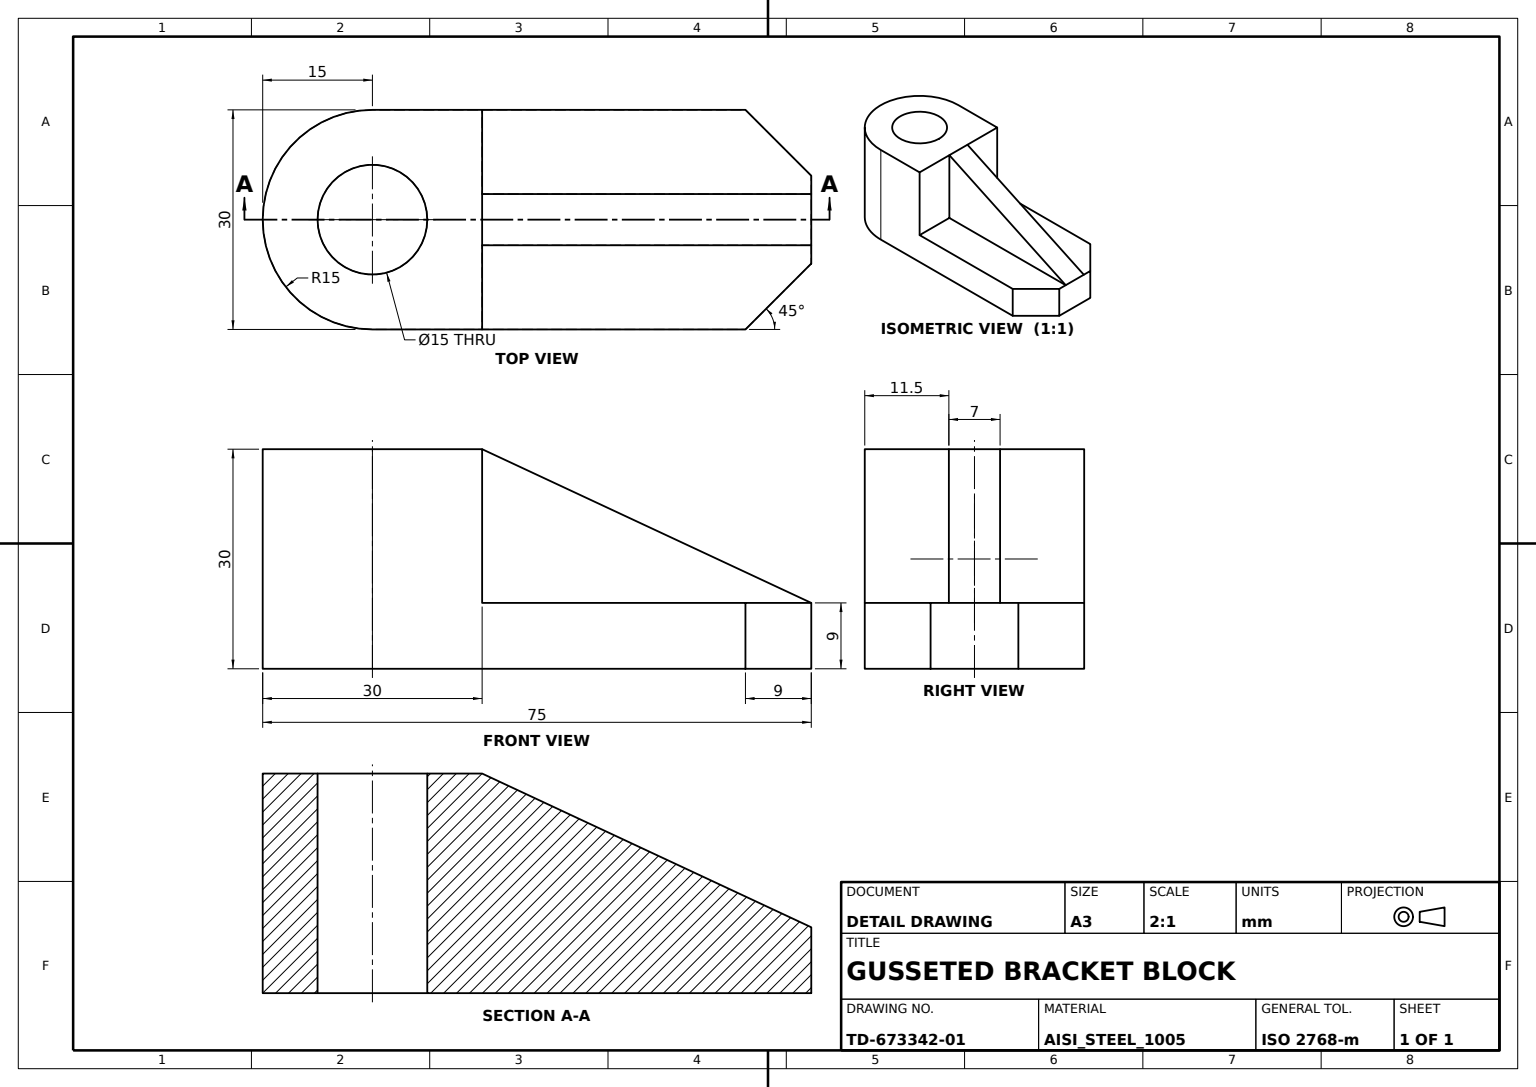
ISO-10303-21;
HEADER;
FILE_DESCRIPTION((''),'2;1');
FILE_NAME('','',(''),(''),'','','');
FILE_SCHEMA(('AUTOMOTIVE_DESIGN'));
ENDSEC;
DATA;
#1=APPLICATION_CONTEXT('');
#2=PRODUCT_CONTEXT('',#1,'mechanical');
#3=PRODUCT('','','',(#2));
#4=PRODUCT_DEFINITION_FORMATION('','',#3);
#5=PRODUCT_DEFINITION_CONTEXT('',#1,'design');
#6=PRODUCT_DEFINITION('','',#4,#5);
#7=PRODUCT_DEFINITION_SHAPE('','',#6);
#8=(LENGTH_UNIT()NAMED_UNIT(*)SI_UNIT(.MILLI.,.METRE.));
#9=(NAMED_UNIT(*)PLANE_ANGLE_UNIT()SI_UNIT($,.RADIAN.));
#10=(NAMED_UNIT(*)SI_UNIT($,.STERADIAN.)SOLID_ANGLE_UNIT());
#11=UNCERTAINTY_MEASURE_WITH_UNIT(LENGTH_MEASURE(0.005),#8,'distance_accuracy_value','');
#12=(GEOMETRIC_REPRESENTATION_CONTEXT(3)GLOBAL_UNCERTAINTY_ASSIGNED_CONTEXT((#11))GLOBAL_UNIT_ASSIGNED_CONTEXT((#8,#9,#10))REPRESENTATION_CONTEXT('',''));
#13=CARTESIAN_POINT('',(6.,75.,9.));
#14=VERTEX_POINT('',#13);
#15=CARTESIAN_POINT('',(6.,75.,0.));
#16=VERTEX_POINT('',#15);
#17=CARTESIAN_POINT('',(6.,75.,24.));
#18=DIRECTION('',(0.,0.,-1.));
#19=VECTOR('',#18,1000.);
#20=LINE('',#17,#19);
#21=EDGE_CURVE('',#14,#16,#20,.T.);
#22=ORIENTED_EDGE('',*,*,#21,.T.);
#23=CARTESIAN_POINT('',(-6.,75.,0.));
#24=VERTEX_POINT('',#23);
#25=CARTESIAN_POINT('',(15.,75.,0.));
#26=DIRECTION('',(-1.,0.,0.));
#27=VECTOR('',#26,1000.);
#28=LINE('',#25,#27);
#29=EDGE_CURVE('',#16,#24,#28,.T.);
#30=ORIENTED_EDGE('',*,*,#29,.T.);
#31=CARTESIAN_POINT('',(-6.,75.,9.));
#32=VERTEX_POINT('',#31);
#33=CARTESIAN_POINT('',(-6.,75.,24.));
#34=LINE('',#33,#19);
#35=EDGE_CURVE('',#32,#24,#34,.T.);
#36=ORIENTED_EDGE('',*,*,#35,.F.);
#37=CARTESIAN_POINT('',(-3.5,75.,9.));
#38=VERTEX_POINT('',#37);
#39=CARTESIAN_POINT('',(15.,75.,9.));
#40=LINE('',#39,#27);
#41=EDGE_CURVE('',#38,#32,#40,.T.);
#42=ORIENTED_EDGE('',*,*,#41,.F.);
#43=CARTESIAN_POINT('',(3.5,75.,9.));
#44=VERTEX_POINT('',#43);
#45=LINE('',#43,#27);
#46=EDGE_CURVE('',#44,#38,#45,.T.);
#47=ORIENTED_EDGE('',*,*,#46,.F.);
#48=EDGE_CURVE('',#14,#44,#40,.T.);
#49=ORIENTED_EDGE('',*,*,#48,.F.);
#50=EDGE_LOOP('',(#22,#30,#36,#42,#47,#49));
#51=FACE_BOUND('',#50,.T.);
#52=DIRECTION('',(0.,-1.,0.));
#53=AXIS2_PLACEMENT_3D('',#25,#52,#18);
#54=PLANE('',#53);
#55=ADVANCED_FACE('',(#51),#54,.F.);
#56=CARTESIAN_POINT('',(15.,66.,9.));
#57=VERTEX_POINT('',#56);
#58=CARTESIAN_POINT('',(10.5,70.5,9.));
#59=DIRECTION('',(0.707106781,-0.707106781,0.));
#60=VECTOR('',#59,1000.);
#61=LINE('',#58,#60);
#62=EDGE_CURVE('',#14,#57,#61,.T.);
#63=ORIENTED_EDGE('',*,*,#62,.T.);
#64=CARTESIAN_POINT('',(15.,66.,0.));
#65=VERTEX_POINT('',#64);
#66=CARTESIAN_POINT('',(15.,66.,24.));
#67=LINE('',#66,#19);
#68=EDGE_CURVE('',#57,#65,#67,.T.);
#69=ORIENTED_EDGE('',*,*,#68,.T.);
#70=CARTESIAN_POINT('',(48.,33.,0.));
#71=DIRECTION('',(-0.707106781,0.707106781,0.));
#72=VECTOR('',#71,1000.);
#73=LINE('',#70,#72);
#74=EDGE_CURVE('',#65,#16,#73,.T.);
#75=ORIENTED_EDGE('',*,*,#74,.T.);
#76=ORIENTED_EDGE('',*,*,#21,.F.);
#77=EDGE_LOOP('',(#63,#69,#75,#76));
#78=FACE_BOUND('',#77,.T.);
#79=DIRECTION('',(0.707106781,0.707106781,0.));
#80=AXIS2_PLACEMENT_3D('',#17,#79,#71);
#81=PLANE('',#80);
#82=ADVANCED_FACE('',(#78),#81,.T.);
#83=CARTESIAN_POINT('',(3.5,30.,9.));
#84=VERTEX_POINT('',#83);
#85=CARTESIAN_POINT('',(3.5,0.,9.));
#86=VECTOR('',#52,1000.);
#87=LINE('',#85,#86);
#88=EDGE_CURVE('',#44,#84,#87,.T.);
#89=ORIENTED_EDGE('',*,*,#88,.F.);
#90=CARTESIAN_POINT('',(3.5,30.,30.));
#91=VERTEX_POINT('',#90);
#92=DIRECTION('',(0.,0.90618314,-0.422885465));
#93=VECTOR('',#92,1000.);
#94=LINE('',#90,#93);
#95=EDGE_CURVE('',#91,#44,#94,.T.);
#96=ORIENTED_EDGE('',*,*,#95,.F.);
#97=CARTESIAN_POINT('',(3.5,30.,0.));
#98=DIRECTION('',(0.,0.,1.));
#99=VECTOR('',#98,1000.);
#100=LINE('',#97,#99);
#101=EDGE_CURVE('',#84,#91,#100,.T.);
#102=ORIENTED_EDGE('',*,*,#101,.F.);
#103=EDGE_LOOP('',(#89,#96,#102));
#104=FACE_BOUND('',#103,.T.);
#105=CARTESIAN_POINT('',(3.5,0.,0.));
#106=AXIS2_PLACEMENT_3D('',#105,#26,#98);
#107=PLANE('',#106);
#108=ADVANCED_FACE('',(#104),#107,.F.);
#109=CARTESIAN_POINT('',(15.,15.,30.));
#110=VERTEX_POINT('',#109);
#111=CARTESIAN_POINT('',(-15.,15.,30.));
#112=VERTEX_POINT('',#111);
#113=CARTESIAN_POINT('',(0.,15.,30.));
#114=DIRECTION('',(0.,1.,0.));
#115=AXIS2_PLACEMENT_3D('',#113,#18,#114);
#116=CIRCLE('',#115,15.);
#117=EDGE_CURVE('',#110,#112,#116,.T.);
#118=ORIENTED_EDGE('',*,*,#117,.T.);
#119=CARTESIAN_POINT('',(-15.,15.,0.));
#120=VERTEX_POINT('',#119);
#121=CARTESIAN_POINT('',(-15.,15.,45.));
#122=LINE('',#121,#19);
#123=EDGE_CURVE('',#112,#120,#122,.T.);
#124=ORIENTED_EDGE('',*,*,#123,.T.);
#125=CARTESIAN_POINT('',(15.,15.,0.));
#126=VERTEX_POINT('',#125);
#127=CARTESIAN_POINT('',(0.,15.,0.));
#128=DIRECTION('',(1.,0.,0.));
#129=AXIS2_PLACEMENT_3D('',#127,#98,#128);
#130=CIRCLE('',#129,15.);
#131=EDGE_CURVE('',#120,#126,#130,.T.);
#132=ORIENTED_EDGE('',*,*,#131,.T.);
#133=CARTESIAN_POINT('',(15.,15.,45.));
#134=LINE('',#133,#19);
#135=EDGE_CURVE('',#110,#126,#134,.T.);
#136=ORIENTED_EDGE('',*,*,#135,.F.);
#137=EDGE_LOOP('',(#118,#124,#132,#136));
#138=FACE_BOUND('',#137,.T.);
#139=CARTESIAN_POINT('',(0.,15.,45.));
#140=AXIS2_PLACEMENT_3D('',#139,#18,#114);
#141=CYLINDRICAL_SURFACE('',#140,15.);
#142=ADVANCED_FACE('',(#138),#141,.T.);
#143=CARTESIAN_POINT('',(0.,22.5,30.));
#144=VERTEX_POINT('',#143);
#145=CIRCLE('',#115,7.5);
#146=EDGE_CURVE('',#144,#144,#145,.F.);
#147=ORIENTED_EDGE('',*,*,#146,.T.);
#148=EDGE_LOOP('',(#147));
#149=FACE_BOUND('',#148,.T.);
#150=CARTESIAN_POINT('',(7.5,15.,0.));
#151=VERTEX_POINT('',#150);
#152=CIRCLE('',#129,7.5);
#153=EDGE_CURVE('',#151,#151,#152,.F.);
#154=ORIENTED_EDGE('',*,*,#153,.T.);
#155=EDGE_LOOP('',(#154));
#156=FACE_BOUND('',#155,.T.);
#157=CYLINDRICAL_SURFACE('',#140,7.5);
#158=ADVANCED_FACE('',(#149,#156),#157,.F.);
#159=CARTESIAN_POINT('',(-15.,66.,9.));
#160=VERTEX_POINT('',#159);
#161=CARTESIAN_POINT('',(-15.,66.,0.));
#162=VERTEX_POINT('',#161);
#163=CARTESIAN_POINT('',(-15.,66.,24.));
#164=LINE('',#163,#19);
#165=EDGE_CURVE('',#160,#162,#164,.T.);
#166=ORIENTED_EDGE('',*,*,#165,.F.);
#167=CARTESIAN_POINT('',(4.5,85.5,9.));
#168=VECTOR('',#79,1000.);
#169=LINE('',#167,#168);
#170=EDGE_CURVE('',#160,#32,#169,.T.);
#171=ORIENTED_EDGE('',*,*,#170,.T.);
#172=ORIENTED_EDGE('',*,*,#35,.T.);
#173=CARTESIAN_POINT('',(-33.,48.,0.));
#174=DIRECTION('',(-0.707106781,-0.707106781,0.));
#175=VECTOR('',#174,1000.);
#176=LINE('',#173,#175);
#177=EDGE_CURVE('',#24,#162,#176,.T.);
#178=ORIENTED_EDGE('',*,*,#177,.T.);
#179=EDGE_LOOP('',(#166,#171,#172,#178));
#180=FACE_BOUND('',#179,.T.);
#181=AXIS2_PLACEMENT_3D('',#163,#71,#174);
#182=PLANE('',#181);
#183=ADVANCED_FACE('',(#180),#182,.T.);
#184=CARTESIAN_POINT('',(15.,30.,9.));
#185=VERTEX_POINT('',#184);
#186=CARTESIAN_POINT('',(15.,30.,30.));
#187=VERTEX_POINT('',#186);
#188=LINE('',#184,#99);
#189=EDGE_CURVE('',#185,#187,#188,.T.);
#190=ORIENTED_EDGE('',*,*,#189,.T.);
#191=LINE('',#186,#86);
#192=EDGE_CURVE('',#187,#110,#191,.T.);
#193=ORIENTED_EDGE('',*,*,#192,.T.);
#194=ORIENTED_EDGE('',*,*,#135,.T.);
#195=CARTESIAN_POINT('',(15.,0.,0.));
#196=VECTOR('',#114,1000.);
#197=LINE('',#195,#196);
#198=EDGE_CURVE('',#126,#65,#197,.T.);
#199=ORIENTED_EDGE('',*,*,#198,.T.);
#200=ORIENTED_EDGE('',*,*,#68,.F.);
#201=LINE('',#39,#86);
#202=EDGE_CURVE('',#57,#185,#201,.T.);
#203=ORIENTED_EDGE('',*,*,#202,.T.);
#204=EDGE_LOOP('',(#190,#193,#194,#199,#200,#203));
#205=FACE_BOUND('',#204,.T.);
#206=AXIS2_PLACEMENT_3D('',#195,#128,#18);
#207=PLANE('',#206);
#208=ADVANCED_FACE('',(#205),#207,.T.);
#209=CARTESIAN_POINT('',(-15.,0.,0.));
#210=LINE('',#209,#196);
#211=EDGE_CURVE('',#120,#162,#210,.T.);
#212=ORIENTED_EDGE('',*,*,#211,.T.);
#213=ORIENTED_EDGE('',*,*,#177,.F.);
#214=ORIENTED_EDGE('',*,*,#29,.F.);
#215=ORIENTED_EDGE('',*,*,#74,.F.);
#216=ORIENTED_EDGE('',*,*,#198,.F.);
#217=ORIENTED_EDGE('',*,*,#131,.F.);
#218=EDGE_LOOP('',(#212,#213,#214,#215,#216,#217));
#219=FACE_BOUND('',#218,.T.);
#220=ORIENTED_EDGE('',*,*,#153,.F.);
#221=EDGE_LOOP('',(#220));
#222=FACE_BOUND('',#221,.T.);
#223=AXIS2_PLACEMENT_3D('',#195,#98,#128);
#224=PLANE('',#223);
#225=ADVANCED_FACE('',(#219,#222),#224,.F.);
#226=ORIENTED_EDGE('',*,*,#146,.F.);
#227=EDGE_LOOP('',(#226));
#228=FACE_BOUND('',#227,.T.);
#229=CARTESIAN_POINT('',(-3.5,30.,30.));
#230=VERTEX_POINT('',#229);
#231=CARTESIAN_POINT('',(-15.,30.,30.));
#232=VERTEX_POINT('',#231);
#233=LINE('',#186,#27);
#234=EDGE_CURVE('',#230,#232,#233,.T.);
#235=ORIENTED_EDGE('',*,*,#234,.T.);
#236=LINE('',#231,#86);
#237=EDGE_CURVE('',#232,#112,#236,.T.);
#238=ORIENTED_EDGE('',*,*,#237,.T.);
#239=ORIENTED_EDGE('',*,*,#117,.F.);
#240=ORIENTED_EDGE('',*,*,#192,.F.);
#241=EDGE_CURVE('',#187,#91,#233,.T.);
#242=ORIENTED_EDGE('',*,*,#241,.T.);
#243=LINE('',#90,#27);
#244=EDGE_CURVE('',#91,#230,#243,.T.);
#245=ORIENTED_EDGE('',*,*,#244,.T.);
#246=EDGE_LOOP('',(#235,#238,#239,#240,#242,#245));
#247=FACE_BOUND('',#246,.T.);
#248=AXIS2_PLACEMENT_3D('',#186,#18,#114);
#249=PLANE('',#248);
#250=ADVANCED_FACE('',(#228,#247),#249,.F.);
#251=ORIENTED_EDGE('',*,*,#46,.T.);
#252=LINE('',#229,#93);
#253=EDGE_CURVE('',#230,#38,#252,.T.);
#254=ORIENTED_EDGE('',*,*,#253,.F.);
#255=ORIENTED_EDGE('',*,*,#244,.F.);
#256=ORIENTED_EDGE('',*,*,#95,.T.);
#257=EDGE_LOOP('',(#251,#254,#255,#256));
#258=FACE_BOUND('',#257,.T.);
#259=DIRECTION('',(0.,0.422885465,0.90618314));
#260=DIRECTION('',(0.,-0.90618314,0.422885465));
#261=AXIS2_PLACEMENT_3D('',#90,#259,#260);
#262=PLANE('',#261);
#263=ADVANCED_FACE('',(#258),#262,.T.);
#264=ORIENTED_EDGE('',*,*,#241,.F.);
#265=ORIENTED_EDGE('',*,*,#189,.F.);
#266=LINE('',#184,#27);
#267=EDGE_CURVE('',#185,#84,#266,.T.);
#268=ORIENTED_EDGE('',*,*,#267,.T.);
#269=ORIENTED_EDGE('',*,*,#101,.T.);
#270=EDGE_LOOP('',(#264,#265,#268,#269));
#271=FACE_BOUND('',#270,.T.);
#272=AXIS2_PLACEMENT_3D('',#184,#52,#18);
#273=PLANE('',#272);
#274=ADVANCED_FACE('',(#271),#273,.F.);
#275=CARTESIAN_POINT('',(-3.5,30.,9.));
#276=VERTEX_POINT('',#275);
#277=CARTESIAN_POINT('',(-3.5,30.,0.));
#278=LINE('',#277,#99);
#279=EDGE_CURVE('',#230,#276,#278,.F.);
#280=ORIENTED_EDGE('',*,*,#279,.F.);
#281=ORIENTED_EDGE('',*,*,#253,.T.);
#282=CARTESIAN_POINT('',(-3.5,0.,9.));
#283=LINE('',#282,#86);
#284=EDGE_CURVE('',#276,#38,#283,.F.);
#285=ORIENTED_EDGE('',*,*,#284,.F.);
#286=EDGE_LOOP('',(#280,#281,#285));
#287=FACE_BOUND('',#286,.T.);
#288=CARTESIAN_POINT('',(-3.5,0.,0.));
#289=AXIS2_PLACEMENT_3D('',#288,#26,#98);
#290=PLANE('',#289);
#291=ADVANCED_FACE('',(#287),#290,.T.);
#292=ORIENTED_EDGE('',*,*,#202,.F.);
#293=ORIENTED_EDGE('',*,*,#62,.F.);
#294=ORIENTED_EDGE('',*,*,#48,.T.);
#295=ORIENTED_EDGE('',*,*,#88,.T.);
#296=ORIENTED_EDGE('',*,*,#267,.F.);
#297=EDGE_LOOP('',(#292,#293,#294,#295,#296));
#298=FACE_BOUND('',#297,.T.);
#299=AXIS2_PLACEMENT_3D('',#39,#18,#114);
#300=PLANE('',#299);
#301=ADVANCED_FACE('',(#298),#300,.F.);
#302=CARTESIAN_POINT('',(-15.,30.,9.));
#303=VERTEX_POINT('',#302);
#304=LINE('',#302,#99);
#305=EDGE_CURVE('',#303,#232,#304,.T.);
#306=ORIENTED_EDGE('',*,*,#305,.F.);
#307=CARTESIAN_POINT('',(-15.,75.,9.));
#308=LINE('',#307,#86);
#309=EDGE_CURVE('',#160,#303,#308,.T.);
#310=ORIENTED_EDGE('',*,*,#309,.F.);
#311=ORIENTED_EDGE('',*,*,#165,.T.);
#312=ORIENTED_EDGE('',*,*,#211,.F.);
#313=ORIENTED_EDGE('',*,*,#123,.F.);
#314=ORIENTED_EDGE('',*,*,#237,.F.);
#315=EDGE_LOOP('',(#306,#310,#311,#312,#313,#314));
#316=FACE_BOUND('',#315,.T.);
#317=AXIS2_PLACEMENT_3D('',#209,#128,#18);
#318=PLANE('',#317);
#319=ADVANCED_FACE('',(#316),#318,.F.);
#320=ORIENTED_EDGE('',*,*,#309,.T.);
#321=EDGE_CURVE('',#276,#303,#266,.T.);
#322=ORIENTED_EDGE('',*,*,#321,.F.);
#323=ORIENTED_EDGE('',*,*,#284,.T.);
#324=ORIENTED_EDGE('',*,*,#41,.T.);
#325=ORIENTED_EDGE('',*,*,#170,.F.);
#326=EDGE_LOOP('',(#320,#322,#323,#324,#325));
#327=FACE_BOUND('',#326,.T.);
#328=ADVANCED_FACE('',(#327),#300,.F.);
#329=ORIENTED_EDGE('',*,*,#279,.T.);
#330=ORIENTED_EDGE('',*,*,#321,.T.);
#331=ORIENTED_EDGE('',*,*,#305,.T.);
#332=ORIENTED_EDGE('',*,*,#234,.F.);
#333=EDGE_LOOP('',(#329,#330,#331,#332));
#334=FACE_BOUND('',#333,.T.);
#335=ADVANCED_FACE('',(#334),#273,.F.);
#336=CLOSED_SHELL('',(#55,#82,#108,#142,#158,#183,#208,#225,#250,#263,#274,#291,#301,#319,#328,#335));
#337=MANIFOLD_SOLID_BREP('',#336);
#338=ADVANCED_BREP_SHAPE_REPRESENTATION('',(#337),#12);
#339=SHAPE_DEFINITION_REPRESENTATION(#7,#338);
ENDSEC;
END-ISO-10303-21;
